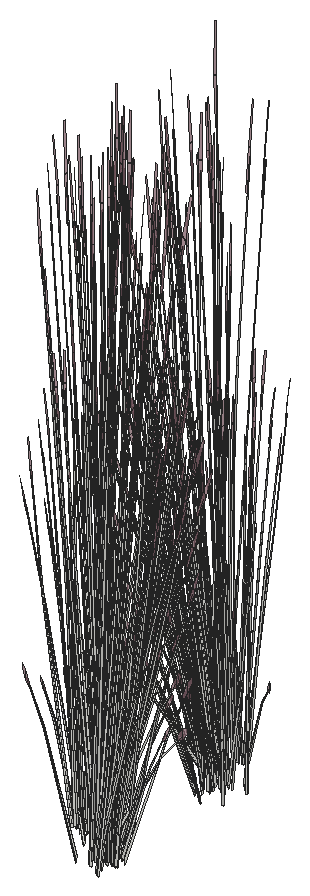
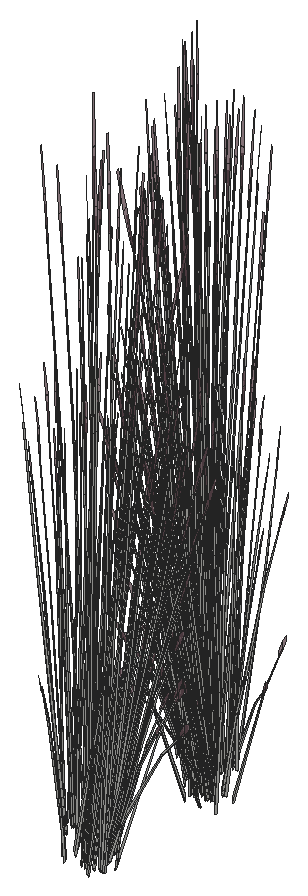
# SketchUp Ruby script. Lengths in inches.
U = 1.inch
M = Sketchup.active_model
def pt(a) = Geom::Point3d.new(a.map { |v| v * U })
def face(e, loops, mat)
  f = e.add_face(loops[0].map { |a| pt(a) })
  loops[1..].each { |l| e.add_face(l.map { |a| pt(a) }).erase! }
  f.material = f.back_material = mat if mat
  f
end
# faces: each face lists its corners as indices into pts; further lists are holes
def faces(e, pts, list, mat = nil) = list.each { |f| face(e, (f[0].is_a?(Array) ? f : [f]).map { |l| l.map { |i| pts[i] } }, mat) }
# xy, xz, yz: faces in a plane at the given z, y or x. An outline is a flat list of corners, or four numbers for a rectangle; further outlines are holes
def ring(l) = l.size == 4 ? [[l[0], l[1]], [l[2], l[1]], [l[2], l[3]], [l[0], l[3]]] : l.each_slice(2).to_a
def flat(e, list, mat, &to3) = list.each { |f| face(e, (f[0].is_a?(Array) ? f : [f]).map { |l| ring(l).map { |u, v| to3.(u, v) } }, mat) }
def xy(e, z, list, mat = nil) = flat(e, list, mat) { |x, y| [x, y, z] }
def xz(e, y, list, mat = nil) = flat(e, list, mat) { |x, z| [x, y, z] }
def yz(e, x, list, mat = nil) = flat(e, list, mat) { |y, z| [x, y, z] }
def lines(e, pts, list) = list.each { |a, b| e.add_line(pt(pts[a]), pt(pts[b])) }
# prism: a flat outline (further loops are holes) pulled along v
def prism(e, loops, v, mat = nil)
  f = face(e, loops, mat); d = Geom::Vector3d.new(v.map { |x| x * U })
  f.pushpull(f.normal.samedirection?(d) ? d.length : -d.length)
end
def box(e, o, s, mat = nil) = prism(e, [[o, [o[0] + s[0], o[1], o[2]], [o[0] + s[0], o[1] + s[1], o[2]], [o[0], o[1] + s[1], o[2]]]], [0, 0, s[2]], mat)
def at(x, y, z, deg = 0) = Geom::Transformation.translation(pt([x, y, z])) * Geom::Transformation.rotation(ORIGIN, Z_AXIS, deg.degrees)
def axes(o, x, y, z) = Geom::Transformation.new([*x, 0, *y, 0, *z, 0, *pt(o).to_a, 1])
def part(name) = M.definitions.add(name)
# library, detail: a bought-in or finely detailed component or shape, given as its bounding box
def library(name, o, s) = part(name).tap { |d| box(d.entities, o, s) }
def detail(e, o, s) = box(e.add_group.entities, o, s)
def put(e, d, t, mat = nil) = e.add_instance(d, t).tap { |i| i.material = mat if mat }
def group(e, t, mat = nil) = e.add_group.tap { |g| g.transformation = t; g.material = mat if mat }.entities
root = M.entities
M.materials.add("LightPink_Translucent").color = [144, 107, 117]
M.materials["LightPink_Translucent"].alpha = 0.75
c1 = part("blade")
p = [[2.15,0.21,22],[0,0.17,0],[0.09,0.45,0],[2.18,0.31,22],[2.29,0.31,22],[0.38,0.45,0],
  [2.48,0.24,33],[2.49,0.24,33],[2.48,0.22,33]]
faces(c1.entities,p,[[0,1,2,3],[4,5,2,3],[6,3,4,7],[8,0,3,6]])
c2 = part("seeds")
p = [[0.3,-0.1,1.38],[-0.01,-0.03,1.59],[-0.01,-0.03,0.03],[0.14,-0.07,-0.07],[0.29,-0.03,3],[0.15,0.01,3.11]]
faces(c2.entities,p,[[0,1,2,3],[1,0,4,5]],"LightPink_Translucent")
c3 = part("blade with seeds")
put(c3.entities,c1,at(0,0,0))
put(c3.entities,c2,axes([2.4,0.25,30.99],[1.5799,-0.05474,1.17369],[-0.12525,1.92788,0.29478],[-0.07173,-0.02425,1.56792]))
put(root,c3,axes([329.36,454.8,1399.49],[0.00895,0.0735,1.76342],[-0.18044,0.38382,-0.26939],[-0.12817,-0.01935,0.30037]))
put(root,c3,axes([331.25,454.39,1400.72],[-0.21202,-0.39143,0.44739],[0.32115,-0.27564,-0.21531],[0.06861,0.04843,1.43643]))
put(root,c3,axes([330.15,456.18,1400.03],[-0.08291,-0.40636,-0.30978],[0.32928,-0.11539,0.30978],[-0.06638,-0.04686,1.38974]))
put(root,c3,axes([330.58,456.16,1400.47],[0.37926,-0.12378,0.17642],[0.09365,0.46065,0.35086],[-0.03382,-0.06712,1.60407]))
put(root,c3,axes([331.36,454.42,1400.67],[0.35635,-0.30962,-0.29095],[0.23697,0.43749,-0.50002],[0.08792,0.04443,1.59708]))
put(root,c3,axes([332.78,455.23,1402.53],[0.29332,0.1301,-0.35414],[-0.08555,0.37955,0.4572],[0.11809,-0.0348,0.87481]))
put(root,c3,axes([330.0625,456.36,1400.02],[-0.33032,-0.23318,-0.49651],[0.19744,-0.41812,0],[-0.07523,-0.05311,1.57504]))
put(root,c3,axes([332.26,453.59,1400.02],[0.33032,0.23318,-0.49651],[-0.19744,0.41812,0],[0.07523,0.05311,1.57504]))
put(root,c3,axes([329.33,454.63,1402.53],[-0.29332,-0.1301,-0.35414],[0.08555,-0.37955,0.4572],[-0.11809,0.0348,0.87481]))
put(root,c3,axes([331.63,454.92,1400.21],[0.39487,0,0],[0,0.48281,0],[0,0,1.78407]))
put(root,c3,axes([330.96,455.53,1400.67],[-0.35635,0.30962,-0.29095],[-0.23697,-0.43749,-0.50002],[-0.08792,-0.04443,1.59708]))
put(root,c3,axes([331.74,453.79,1400.47],[-0.37926,0.12378,0.17642],[-0.09365,-0.46065,0.35086],[0.03382,0.06712,1.60407]))
put(root,c3,axes([331.98,454.76,1401.875],[-0.14639,0.01056,1.71376],[0.09712,-0.45778,0.13857],[0.20862,0.02831,0.73262]))
put(root,c3,axes([332.17,453.77,1400.03],[0.08291,0.40636,-0.30978],[-0.32928,0.11539,0.30978],[0.06638,0.04686,1.38974]))
put(root,c3,axes([332.73,455.39,1402.73],[0.12963,0.31798,0.0643],[-0.23638,0.15564,0.50621],[0.1042,-0.03071,0.77189]))
put(root,c3,axes([331.5,454.68,1400.38],[-0.44609,-0.09826,0.49198],[0.09078,-0.55493,0.19306],[0.06519,0.05359,1.70813]))
put(root,c3,axes([332.71,455.28,1402.73],[-0.09971,0.42522,0.48003],[-0.32782,-0.1454,0.3958],[0.12892,-0.02555,0.9933]))
put(root,c3,axes([331.15,456.05,1400.2],[-0.11516,-0.40207,0],[0.32884,-0.1408,0],[0,0,1.54371]))
put(root,c3,axes([330.93,455.67,1400.62],[-0.06809,0.4162,0.1448],[-0.33266,-0.07225,-0.41347],[-0.06054,-0.04274,1.26744]))
put(root,c3,axes([329.64,454.59,1403.05],[0.29332,0.1301,0.35414],[-0.08555,0.37955,-0.4572],[-0.11809,0.0348,0.87481]))
put(root,c3,axes([331.58,455.99,1400.18],[0.37054,-0.15823,-0.19198],[0.1302,0.45581,0.00008],[0.0409,-0.01749,1.73897]))
put(root,c3,axes([331.71,456.18,1400.47],[0.10196,-0.46348,0.17642],[0.3731,0.13116,0.35086],[-0.06445,0.00226,1.60407]))
put(root,c3,axes([331.62,455.13,1400.21],[0.24637,0.30123,0],[-0.24637,0.30123,0],[0,0,1.69266]))
put(root,c3,axes([330.22,454.57,1401.34],[0.10032,-0.06746,1.77064],[0.0346,0.47103,0.13857],[-0.2173,0.0625,0.63284]))
put(root,c3,axes([332.29,455,1400.47],[-0.2773,-0.3397,0.17642],[0.27945,-0.32949,0.35086],[-0.03063,0.06937,1.60407]))
put(root,c3,axes([331.78,454.49,1400.06],[0.36714,0.07646,-0.62353],[-0.07747,0.47163,-0.16365],[0.10956,0.05715,1.37633]))
put(root,c3,axes([333.4,455.3125,1400.77],[-0.21807,0.07699,1.1486],[0.10265,-0.31819,0.84392],[0.11568,0.02177,0.25299]))
put(root,c3,axes([331.07,456.23,1400.2],[-0.35581,-0.20937,0],[0.17124,-0.43505,0],[0,0,1.62707]))
put(root,c3,axes([331.36,455.67,1400.46],[-0.34464,-0.37536,-0.25192],[0.29,-0.42149,0.5513],[-0.0928,0.04391,1.68216]))
put(root,c3,axes([330.45,456.39,1400.48],[0.33032,0.23318,0.49651],[-0.19744,0.41812,0],[-0.07523,-0.05311,1.57504]))
put(root,c3,axes([331.62,454.78,1400.72],[0.17124,-0.42022,0.44739],[0.35581,0.20224,-0.21531],[0,0.09687,1.43643]))
put(root,c3,axes([333.3,456.66,1402.71],[-0.03191,-0.04083,1.77383],[0.06981,-0.43764,-0.16761],[0.12571,-0.02796,0.31391]))
put(root,c3,axes([329.14,454.88,1402.72],[-0.05763,0.06055,1.74944],[0.0049,0.44239,-0.27667],[-0.13211,0.05753,0.14031]))
put(root,c3,axes([331.55,455.02,1400.29],[0,0.53934,-0.05637],[-0.44133,0,0],[0,0.01695,1.79368]))
put(root,c3,axes([329.53,454.82,1402.68],[-0.09562,0.42421,-0.51099],[-0.32782,-0.1454,-0.3958],[-0.13199,0.0389,0.97773]))
put(root,c3,axes([329.51,454.46,1403.03],[0.17758,0.42229,-0.1216],[-0.31518,0.20752,-0.67495],[-0.13282,0.05572,1.02557]))
put(root,c3,axes([331.58,454.64,1400.21],[0.21202,0.39143,-0.44739],[-0.32115,0.27564,0.21531],[0.06861,0.04843,1.43643]))
put(root,c3,axes([333.02,456.29,1401.93],[-0.06755,-0.39203,-0.03492],[0.31928,-0.09013,-0.15832],[0.06667,0.02485,0.52218]))
put(root,c3,axes([330.26,456.64,1400.375],[-0.22066,0.46731,0],[-0.36918,-0.26061,-0.51607],[-0.08408,-0.05936,1.63711]))
put(root,c3,axes([332.19,456.28,1403.03],[0.0189,-0.47427,-0.1216],[0.35781,0.01296,-0.67495],[0.13781,0.03295,1.02557]))
put(root,c3,axes([332.52,455.01,1400.48],[0,-0.46636,0.49651],[0.39487,0,0],[0,0.10622,1.57504]))
put(root,c3,axes([331.53,455.36,1400.72],[0.38326,-0.02879,0.44739],[0.03466,0.47788,-0.21531],[-0.06861,0.04843,1.43643]))
put(root,c3,axes([331.77,454.875,1400.62],[0.32884,-0.136,0.1448],[0.11516,0.38837,-0.41347],[0,0.08547,1.26744]))
put(root,c3,axes([332.14,456.09,1403.05],[-0.20082,-0.29199,0.35414],[0.2293,-0.2764,-0.4572],[0.1165,0.04206,0.87481]))
put(root,c3,axes([331.1875,455.59,1400.21],[-0.38326,0.02879,-0.44739],[-0.03466,-0.47788,0.21531],[-0.06861,0.04843,1.43643]))
put(root,c3,axes([332.99,455.82,1400.59],[-0.085,-0.1147,1.43002],[0.1106,-0.37943,-0.30754],[0.17198,0.0514,0.61141]))
put(root,c3,axes([331.47,456.24,1400.2],[0.35581,0.20937,0],[-0.17124,0.43505,0],[0,0,1.74954]))
put(root,c3,axes([332.5,456,1402.72],[0.07571,-0.00789,1.74944],[0.20767,-0.36231,-0.27667],[0.13467,0.04783,0.14031]))
put(root,c3,axes([331.61,456.7,1400.19],[-0.21791,-0.46895,-0.05142],[0.36918,-0.26061,0.51607],[-0.09097,0.04465,1.6363]))
put(root,c3,axes([331.53,455.57,1400.62],[0.26075,0.2802,0.1448],[-0.2175,0.31612,-0.41347],[-0.06054,0.04274,1.26744]))
put(root,c3,axes([329.47,455.64,1402.73],[-0.08753,-0.42921,0.48003],[0.34336,-0.07449,0.3958],[-0.1012,0.10094,0.9933]))
put(root,c3,axes([329.41,455.56,1402.73],[-0.2423,-0.19613,0.0643],[0.14107,-0.2793,0.50621],[-0.07768,0.0903,0.77189]))
put(root,c3,axes([329.52,455.04,1401.875],[0.12246,-0.09864,1.71376],[0.1031,0.45582,0.13857],[-0.19225,0.10302,0.73262]))
put(root,c3,axes([332.21,456.05,1402.98],[0.35281,0.01123,-0.71045],[-0.0237,0.47284,0.08574],[0.14947,0.0499,1.00501]))
put(root,c3,axes([331.8125,456.43,1400.48],[0.33032,-0.23318,0.49651],[0.19744,0.41812,0],[-0.07523,0.05311,1.57504]))
put(root,c3,axes([331.34,456.0625,1400.29],[0.15345,0.53576,-0.06012],[-0.43845,0.18773,0],[0.00536,0.01871,1.72173]))
put(root,c3,axes([331.51,456.64,1400.03],[-0.32928,-0.11539,-0.30978],[0.08291,-0.40636,0.30978],[-0.06638,0.04686,1.38974]))
put(root,c3,axes([329.14,455.82,1400.59],[0.12266,0.03828,1.43002],[0.07906,0.39104,-0.30754],[-0.16661,0.0732,0.61141]))
put(root,c3,axes([329.6875,455.5,1403.05],[0.30722,-0.06665,0.35414],[0.08112,0.381,-0.4572],[-0.08804,0.10234,0.87481]))
put(root,c3,axes([332.78,455.09,1400.375],[0.44133,0,0],[0,0.52122,-0.51607],[0,0.11871,1.63711]))
put(root,c3,axes([328.5,455.33,1402.71],[0.04504,0.01251,1.77383],[0.13934,0.41205,-0.16761],[-0.0922,0.10815,0.31391]))
put(root,c3,axes([332.61,455.36,1400.2],[-0.44111,-0.00373,-0.04976],[0,-0.52122,0.49943],[-0.01386,0.11865,1.58352]))
put(root,c3,axes([331.65,454.91,1400.67],[0.39748,0.22252,-0.29095],[-0.19139,0.46966,-0.50002],[0.01249,0.11531,1.59708]))
put(root,c3,axes([328.88,456.64,1400.77],[0.14709,-0.21136,1.1486],[0.05804,0.3346,0.84392],[-0.1063,0.05991,0.25299]))
put(root,c3,axes([332.42,456.25,1402.53],[0.20082,0.29199,-0.35414],[-0.2293,0.2764,0.4572],[0.1165,0.04206,0.87481]))
put(root,c3,axes([332.52,455.4375,1400.03],[-0.24637,0.29097,-0.30978],[-0.24637,-0.29097,0.30978],[0,0.09372,1.38974]))
put(root,c3,axes([331.46,455.46,1400.67],[0.04113,0.53214,-0.29095],[-0.42835,0.03218,-0.50002],[-0.07543,0.07088,1.59708]))
put(root,c3,axes([332.32,456.36,1402.73],[-0.01777,0.35463,0.0643],[-0.26836,-0.00972,0.50621],[0.1028,0.03711,0.77189]))
put(root,c3,axes([331.61,455.26,1400.21],[-0.17124,0.42022,-0.44739],[-0.35581,-0.20224,0.21531],[0,0.09687,1.43643]))
put(root,c3,axes([329.43,455.72,1402.53],[-0.30722,0.06665,-0.35414],[-0.08112,-0.381,0.4572],[-0.08804,0.10234,0.87481]))
put(root,c3,axes([332.34,456.25,1402.73],[-0.26024,0.30729,0.48003],[-0.22444,-0.32634,0.3958],[0.1221,0.05668,0.9933]))
put(root,c3,axes([328.99,456.58,1403.65],[0.31145,0.12449,-0.06488],[-0.0958,0.38314,-0.29416],[-0.05094,0.05817,0.97024]))
put(root,c3,axes([331.2,455.87,1400.06],[-0.23773,0.35053,-0.62353],[-0.29532,-0.31785,-0.16365],[-0.09526,0.08744,1.37633]))
put(root,c3,axes([331.52,456.6,1403.05],[-0.05451,-0.37564,0.35414],[0.31161,-0.09919,-0.4572],[0.0837,0.10765,0.87481]))
put(root,c3,axes([331.62,456.46,1400.33],[0.44186,0.15158,0.30756],[-0.11054,0.54181,-0.36492],[-0.07313,0.06781,1.64885]))
put(root,c3,axes([331.59,456.83,1400.02],[-0.33032,0.23318,-0.49651],[-0.19744,-0.41812,0],[-0.07523,0.05311,1.57504]))
put(root,c3,axes([332.6875,455.45,1400.02],[0,0.46636,-0.49651],[-0.39487,0,0],[0,0.10622,1.57504]))
put(root,c3,axes([331.7,455.5,1401.875],[-0.1311,-0.08035,1.71376],[0.27131,-0.33708,0.13857],[0.16909,0.15206,0.73262]))
put(root,c3,axes([331.72,454.44,1402.47],[-0.30498,-0.24231,1.38283],[0.32203,-0.37727,0.59665],[0.0984,0.22736,1.33663]))
put(root,c3,axes([329.53,455.46,1403.03],[0.32648,0.25715,-0.1216],[-0.18809,0.3724,-0.67495],[-0.09224,0.12945,1.02557]))
put(root,c3,axes([332.18,456.41,1400.77],[-0.19872,-0.13409,1.1486],[0.2566,-0.13625,0.84392],[0.06921,0.11541,0.25299]))
put(root,c3,axes([331.49,456.8,1403.03],[0.21031,-0.39918,-0.1216],[0.30457,0.22997,-0.67495],[0.10587,0.11278,1.02557]))
put(root,c3,axes([329.97,455.35,1401.875],[0.08815,-0.14329,1.71376],[0.22258,0.38678,0.13857],[-0.15267,0.17614,0.73262]))
put(root,c3,axes([329.6875,455.77,1402.68],[0.09067,0.42583,-0.51099],[-0.34336,0.07449,-0.3958],[-0.0984,0.11438,0.97773]))
put(root,c3,axes([330.1,456.26,1403.05],[0.23881,-0.24554,0.35414],[0.22606,0.28036,-0.4572],[-0.0344,0.14245,0.87481]))
put(root,c3,axes([331.89,456.75,1400.375],[0.22066,0.46731,0],[-0.36918,0.26061,-0.51607],[-0.08408,0.05936,1.63711]))
put(root,c3,axes([331.21,457.13,1402.71],[0.00104,-0.05646,1.77383],[0.30246,-0.2491,-0.16761],[0.10506,0.08891,0.31391]))
put(root,c3,axes([332.24,456.91,1399.49],[0.02571,-0.06733,1.76342],[0.32373,-0.19829,-0.26939],[0.09815,0.10263,0.30037]))
put(root,c3,axes([331.7,454.9,1400.84],[-0.00964,-0.43909,1.41272],[0.43635,0.11382,0.59816],[-0.1032,0.24027,1.3335]))
put(root,c3,axes([331.8125,455.38,1400.09],[0.12941,0.42699,-0.69212],[-0.37279,0.15378,-0.18165],[0.0143,0.14459,1.52773]))
put(root,c3,axes([329.88,456.48,1402.73],[-0.29004,-0.02173,0.0643],[0.00795,-0.32812,0.50621],[-0.03035,0.12569,0.77189]))
put(root,c3,axes([329.27,456.85,1399.49],[0.04734,0.04659,1.76342],[0.08027,0.4317,-0.26939],[-0.10492,0.09206,0.30037]))
put(root,c3,axes([329.98,456.51,1402.73],[-0.25132,-0.3182,0.48003],[0.2669,-0.27442,0.3958],[-0.04636,0.14929,0.9933]))
put(root,c3,axes([331.74,456.6,1402.68],[0.34827,-0.11086,-0.51099],[0.06092,0.41983,-0.3958],[0.09354,0.12031,0.97773]))
put(root,c3,axes([330.77,456.66,1403.05],[0.1064,-0.35863,0.35414],[0.31043,0.1046,-0.4572],[0.02846,0.14439,0.87481]))
put(root,c3,axes([332.22,457.02,1400.67],[-0.22633,-0.01463,1.0506],[0.14947,-0.31064,0.58006],[0.08941,0.11036,0.8241]))
put(root,c3,axes([331.56,456.94,1402.73],[-0.16041,0.29625,0.0643],[-0.22843,-0.17248,0.50621],[0.07385,0.09498,0.77189]))
put(root,c3,axes([331.1875,457.94,1403.65],[0.2439,-0.26754,-0.06488],[0.22348,0.29302,-0.29416],[0.01573,0.08303,0.97024]))
put(root,c3,axes([331.63,456.86,1402.73],[-0.35104,0.10702,0.48003],[-0.06092,-0.41983,0.3958],[0.08256,0.12373,0.9933]))
put(root,c3,axes([329.9,455.7,1401.875],[0.06572,-0.16029,1.71376],[0.27569,0.33172,0.13857],[-0.12437,0.20675,0.73262]))
put(root,c3,axes([331.48,456.27,1400.59],[0.00623,-0.15459,1.43002],[0.29764,-0.17268,-0.30754],[0.09188,0.18503,0.61141]))
put(root,c3,axes([330.67,456.99,1402.73],[-0.26007,0.1585,0.0643],[-0.12729,-0.28902,0.50621],[0.02512,0.1274,0.77189]))
put(root,c3,axes([329.98,456.61,1402.53],[-0.23881,0.24554,-0.35414],[-0.22606,-0.28036,0.4572],[-0.0344,0.14245,0.87481]))
put(root,c3,axes([329.15,456.53,1402.72],[-0.00877,0.09229,1.74944],[0.24897,0.32105,-0.27667],[-0.06518,0.15182,0.14031]))
put(root,c3,axes([329.95,456.32,1403.4],[0.3879,0.02311,-0.13498],[-0.0106,0.43749,-0.74919],[-0.02694,0.1685,1.13838]))
put(root,c3,axes([330.67,456.8125,1403.03],[0.34538,-0.21713,-0.1216],[0.16972,0.38536,-0.67495],[0.04557,0.16239,1.02557]))
put(root,c3,axes([330.77,456.96,1403.0625],[-0.34777,-0.12192,0.53283],[0.11892,-0.40083,0.43934],[0.0209,0.15763,1.10256]))
put(root,c3,axes([330.13,457.56,1400.77],[-0.00913,-0.2773,1.1486],[0.22824,0.19778,0.84392],[-0.04489,0.13217,0.25299]))
put(root,c3,axes([330.73,456.9,1399.49],[0.05712,-0.02538,1.76342],[0.34359,0.13968,-0.26939],[0.01005,0.15742,0.30037]))
put(root,c3,axes([330.21,456.49,1403],[0.25266,0.31335,-0.5672],[-0.2669,0.27442,-0.43934],[-0.03844,0.15921,1.08528]))
put(root,c3,axes([329.9375,456.96,1400.82],[0.32063,-0.08258,0.06507],[0.07371,0.33271,-0.86304],[-0.02033,0.16842,0.7736]))
put(root,c3,axes([330.96,456.79,1402.68],[0.34695,0.11691,-0.51099],[-0.11892,0.40083,-0.3958],[0.03181,0.16138,0.97773]))
put(root,c3,axes([331.16,455.97,1401.875],[-0.08068,-0.14973,1.71376],[0.3728,-0.12606,0.13857],[0.08426,0.23506,0.73262]))
put(root,c3,axes([330.8,457.04,1402.53],[-0.1064,0.35863,-0.35414],[-0.31043,-0.1046,0.4572],[0.02846,0.14439,0.87481]))
put(root,c3,axes([330.13,456.35,1403.34],[-0.00918,0.43138,-0.7886],[-0.38672,-0.02897,0.09517],[-0.04081,0.18275,1.11556]))
put(root,c3,axes([329.125,457.48,1402.71],[0.04004,-0.02816,1.77383],[0.33095,0.18728,-0.16761],[-0.00778,0.15594,0.31391]))
put(root,c3,axes([330.5,456.04,1401.875],[-0.00864,-0.17899,1.71376],[0.37441,0.11874,0.13857],[-0.02316,0.25508,0.73262]))
put(root,c3,axes([330.84,456.72,1402.98],[0.16845,0.3792,-0.71045],[-0.34676,0.21133,0.08574],[0.03939,0.18322,1.00501]))
put(root,c3,axes([329.86,457.3125,1400.59],[0.11138,-0.07357,1.43002],[0.27499,0.22183,-0.30754],[-0.08185,0.19194,0.61141]))
put(root,c3,axes([330.58,457.67,1402.72],[0.04474,0.0751,1.74944],[0.36104,0.0295,-0.27667],[0.03631,0.16562,0.14031]))
put(root,c3,axes([330.01,456.95,1401.36],[0.00775,-0.24075,1.54345],[0.34877,0.12716,0.21329],[-0.03022,0.25658,0.72882]))
put(root,c3,axes([330.27,468.32,1401.875],[0.08068,0.14973,1.71376],[-0.3728,0.12606,0.13857],[-0.08426,-0.23506,0.73262]))
put(root,c3,axes([330.89,467.32,1402.72],[-0.05398,-0.06539,1.74944],[-0.36026,0.04145,-0.27667],[-0.0575,-0.15639,0.14031]))
put(root,c3,axes([331.72,468.1,1400.59],[-0.10032,0.0944,1.43002],[-0.30046,-0.16522,-0.30754],[0.05569,-0.20547,0.61141]))
put(root,c3,axes([331.27,468.43,1402.98],[-0.16845,-0.3792,-0.71045],[0.34676,-0.21133,0.08574],[-0.03939,-0.18322,1.00501]))
put(root,c3,axes([330.17,467.92,1400.59],[-0.02137,0.15256,1.43002],[-0.31245,0.12771,-0.30754],[-0.07303,-0.19719,0.61141]))
put(root,c3,axes([330.98,467.59,1399.49],[-0.0592,0.0168,1.76342],[-0.32738,-0.18913,-0.26939],[0.00549,-0.15776,0.30037]))
put(root,c3,axes([331.97,468.8,1402.98],[0.00918,-0.43138,-0.71045],[0.38672,0.02897,0.08574],[0.04081,-0.18275,1.00501]))
put(root,c3,axes([332.51,468.125,1402.72],[-0.00341,-0.09282,1.74944],[-0.28775,-0.26825,-0.27667],[0.04449,-0.16261,0.14031]))
put(root,c3,axes([331.3,468.11,1402.53],[0.1064,-0.35863,-0.35414],[0.31043,0.1046,0.4572],[-0.02846,-0.14439,0.87481]))
put(root,c3,axes([331.53,468.58,1401.875],[-0.06572,0.16029,1.71376],[-0.27569,-0.33172,0.13857],[0.12437,-0.20675,0.73262]))
put(root,c3,axes([332.43,467.79,1402.71],[-0.03584,0.03562,1.77383],[-0.35118,-0.12018,-0.16761],[-0.01271,-0.15545,0.31391]))
put(root,c3,axes([331.14,468.35,1402.68],[-0.34695,-0.11691,-0.51099],[0.11892,-0.40083,-0.3958],[-0.03181,-0.16138,0.97773]))
put(root,c3,axes([331.35,467.35,1400.77],[0.04528,0.27194,1.1486],[-0.25117,-0.15062,0.84392],[0.02703,-0.13924,0.25299]))
put(root,c3,axes([331.89,468.66,1402.68],[-0.25266,-0.31335,-0.51099],[0.2669,-0.27442,-0.3958],[0.03844,-0.15921,0.97773]))
put(root,c3,axes([330.52,467.11,1402.71],[-0.00658,0.0559,1.77383],[-0.32474,0.20287,-0.16761],[-0.09556,-0.1037,0.31391]))
put(root,c3,axes([330.45,468.1,1403.09],[0.39316,-0.11987,0.53763],[0.06823,0.47021,0.4433],[-0.09247,-0.13858,1.11249]))
put(root,c3,axes([331.34,468.19,1402.73],[0.34777,0.12192,0.48003],[-0.11892,0.40083,0.3958],[-0.0209,-0.15763,0.9933]))
put(root,c3,axes([331.4375,468.33,1403.03],[-0.34538,0.21713,-0.1216],[-0.16972,-0.38536,-0.67495],[-0.04557,-0.16239,1.02557]))
put(root,c3,axes([332.15,468.82,1403.03],[-0.3879,-0.02311,-0.1216],[0.0106,-0.43749,-0.67495],[0.02694,-0.1685,1.02557]))
put(root,c3,axes([332.13,468.54,1402.53],[0.23881,-0.24554,-0.35414],[0.22606,0.28036,0.4572],[0.0344,-0.14245,0.87481]))
put(root,c3,axes([330.0625,467.68,1400.77],[0.18411,0.16231,1.1486],[-0.26813,0.09757,0.84392],[-0.05737,-0.12474,0.25299]))
put(root,c3,axes([331.43,468.16,1402.73],[0.26007,-0.1585,0.0643],[0.12729,0.28902,0.50621],[-0.02512,-0.1274,0.77189]))
put(root,c3,axes([330.51,468.54,1402.98],[-0.30095,-0.22541,-0.71045],[0.21388,-0.395,0.08574],[-0.10904,-0.13459,1.00501]))
put(root,c3,axes([330.4,468.24,1402.53],[-0.05451,-0.37564,-0.35414],[0.31161,-0.09919,0.4572],[-0.0837,-0.10765,0.87481]))
put(root,c3,axes([330.54,468.2,1402.73],[0.16041,-0.29625,0.0643],[0.22843,0.17248,0.50621],[-0.07385,-0.09498,0.77189]))
put(root,c3,axes([329.92,468.16,1399.49],[-0.03419,0.06144,1.76342],[-0.3455,0.13246,-0.26939],[-0.08346,-0.12049,0.30037]))
put(root,c3,axes([330.49,469.85,1400.1],[-0.14494,-0.47823,-0.69835],[0.41752,-0.17223,-0.18329],[-0.01602,-0.16194,1.54149]))
put(root,c3,axes([329.73,468.78,1401.875],[0.1311,0.08035,1.71376],[-0.27131,0.33708,0.13857],[-0.16909,-0.15206,0.73262]))
put(root,c3,axes([332.43,468.39,1399.49],[-0.05283,-0.03674,1.76342],[-0.13569,-0.41045,-0.26939],[0.09154,-0.11138,0.30037]))
put(root,c3,axes([331.33,468.48,1403.05],[-0.1064,0.35863,0.35414],[-0.31043,-0.1046,-0.4572],[-0.02846,-0.14439,0.87481]))
put(root,c3,axes([330.37,468.55,1402.68],[-0.34827,0.11086,-0.51099],[-0.06092,-0.41983,-0.3958],[-0.09354,-0.12031,0.97773]))
put(root,c3,axes([332.125,468.64,1402.73],[0.25132,0.3182,0.48003],[-0.2669,0.27442,0.3958],[0.04636,-0.14929,0.9933]))
put(root,c3,axes([330.61,468.17,1403.43],[-0.23555,0.44708,-0.13619],[-0.34112,-0.25757,-0.75594],[-0.11858,-0.12631,1.14864]))
put(root,c3,axes([332.22,468.67,1402.73],[0.29004,0.02173,0.0643],[-0.00795,0.32812,0.50621],[0.03035,-0.12569,0.77189]))
put(root,c3,axes([332,468.89,1403.05],[-0.23881,0.24554,0.35414],[-0.22606,-0.28036,-0.4572],[0.0344,-0.14245,0.87481]))
put(root,c3,axes([332.42,469.55,1402.98],[0.18436,-0.36797,-0.71045],[0.32306,0.26151,0.08574],[0.11008,-0.13332,1.00501]))
put(root,c3,axes([330.43,468.48,1400.375],[-0.22066,-0.46731,0],[0.36918,-0.26061,-0.51607],[0.08408,-0.05936,1.63711]))
put(root,c3,axes([332.41,469.38,1402.68],[-0.09067,-0.42583,-0.51099],[0.34336,-0.07449,-0.3958],[0.0984,-0.11438,0.97773]))
put(root,c3,axes([330.92,467.91,1400.13],[-0.2439,0.26754,-0.03893],[-0.22348,-0.29302,-0.17649],[-0.01573,-0.08303,0.58215]))
put(root,c3,axes([329.71,468.04,1402.72],[-0.07594,-0.00329,1.74944],[-0.24177,0.32918,-0.27667],[-0.129,-0.06726,0.14031]))
put(root,c3,axes([332.58,469.68,1403.03],[-0.32648,-0.25715,-0.1216],[0.18809,-0.3724,-0.67495],[0.09224,-0.12945,1.02557]))
put(root,c3,axes([331.23,471.09,1401.33],[0.305,0.18805,1.51261],[-0.29879,0.40513,0.59816],[-0.13384,-0.24012,1.26806]))
put(root,c3,axes([330.59,468.54,1403.05],[0.05451,0.37564,0.35414],[-0.31161,0.09919,-0.4572],[-0.0837,-0.10765,0.87481]))
put(root,c3,axes([329.63,469.79,1400.02],[0,-0.46636,-0.49651],[0.39487,0,0],[0,-0.10622,1.57504]))
put(root,c3,axes([330.73,468.41,1400.02],[0.33032,-0.23318,-0.49651],[0.19744,0.41812,0],[0.07523,-0.05311,1.57504]))
put(root,c3,axes([332.69,469.21,1400.59],[-0.12609,-0.01381,1.43002],[-0.12917,-0.37055,-0.30754],[0.1549,-0.10482,0.61141]))
put(root,c3,axes([329.65,468.79,1403.09],[0.29147,-0.34417,0.53763],[0.25138,0.3655,0.4433],[-0.13675,-0.06349,1.11249]))
put(root,c3,axes([333.38,469.57,1402.71],[-0.0461,-0.00354,1.77383],[-0.19143,-0.37951,-0.16761],[0.07688,-0.12478,0.31391]))
put(root,c3,axes([331.12,469.36,1400.06],[0.23773,-0.35053,-0.62353],[0.29532,0.31785,-0.16365],[0.09526,-0.08744,1.37633]))
put(root,c3,axes([332.84,468.53,1400.77],[-0.11756,0.2374,1.1486],[-0.10105,-0.31895,0.84392],[0.09709,-0.07992,0.25299]))
put(root,c3,axes([332.67,469.42,1402.53],[0.30722,-0.06665,-0.35414],[0.08112,0.381,0.4572],[0.08804,-0.10234,0.87481]))
put(root,c3,axes([329.78,468.79,1402.73],[0.01777,-0.35463,0.0643],[0.26836,0.00972,0.50621],[-0.1028,-0.03711,0.77189]))
put(root,c3,axes([330.71,469.98,1400.21],[0.17124,-0.42022,-0.44739],[0.35581,0.20224,0.21531],[0,-0.09687,1.43643]))
put(root,c3,axes([329.68,468.9,1402.53],[-0.20082,-0.29199,-0.35414],[0.2293,-0.2764,0.4572],[-0.1165,-0.04206,0.87481]))
put(root,c3,axes([330.86,469.77,1400.67],[-0.04113,-0.53214,-0.29095],[0.42835,-0.03218,-0.50002],[0.07543,-0.07088,1.59708]))
put(root,c3,axes([329.8,469.8,1400.03],[0.24637,-0.29097,-0.30978],[0.24637,0.29097,0.30978],[0,-0.09372,1.38974]))
put(root,c3,axes([329.7,468.4,1400.13],[-0.10181,0.3808,-0.03893],[-0.31336,-0.11714,-0.17649],[-0.04758,-0.06228,0.58215]))
put(root,c3,axes([332.42,469.65,1403.05],[-0.30722,0.06665,0.35414],[-0.08112,-0.381,-0.4572],[0.08804,-0.10234,0.87481]))
put(root,c3,axes([330.67,470.33,1400.67],[-0.39748,-0.22252,-0.29095],[0.19139,-0.46966,-0.50002],[-0.01249,-0.11531,1.59708]))
put(root,c3,axes([329.53,470.14,1400.375],[-0.44133,0,0],[0,-0.52122,-0.51607],[0,-0.11871,1.63711]))
put(root,c3,axes([329.61,469.21,1400.59],[0.06891,0.12984,1.43002],[-0.15879,0.35293,-0.30754],[-0.16304,-0.08436,0.61141]))
put(root,c3,axes([330.81,468.59,1400.03],[0.32928,0.11539,-0.30978],[-0.08291,0.40636,0.30978],[0.06638,-0.04686,1.38974]))
put(root,c3,axes([329.89,469.09,1402.98],[-0.35281,-0.01123,-0.71045],[0.0237,-0.47284,0.08574],[-0.14947,-0.0499,1.00501]))
put(root,c3,axes([332.7,469.59,1402.73],[0.2423,0.19613,0.0643],[-0.14107,0.2793,0.50621],[0.07768,-0.0903,0.77189]))
put(root,c3,axes([332.63,469.5,1402.73],[0.08753,0.42921,0.48003],[-0.34336,0.07449,0.3958],[0.1012,-0.10094,0.9933]))
put(root,c3,axes([333.55,470.02,1402.72],[0.04898,-0.07104,1.74944],[-0.06269,-0.43574,-0.27667],[0.12289,-0.08262,0.14031]))
put(root,c3,axes([329.875,470,1400.33],[-0.32829,0.39208,0.30756],[-0.32849,-0.38796,-0.36492],[-0.01146,-0.11134,1.64885]))
put(root,c3,axes([329.42,468.32,1402.71],[0.02617,0.04654,1.77383],[-0.12614,0.41836,-0.16761],[-0.12775,0.00303,0.31391]))
put(root,c3,axes([330.92,470.19,1400.43],[0.39767,0.22603,0.24065],[-0.19139,0.46966,0.50002],[0,-0.10827,1.60543]))
put(root,c3,axes([330.77,470.82,1400.4375],[0.09355,-0.55261,-0.23429],[0.44354,0.09633,0.51271],[-0.0775,-0.07631,1.5644]))
put(root,c3,axes([329.78,469.1875,1402.68],[-0.25628,0.30892,-0.51099],[-0.22444,-0.32634,-0.3958],[-0.13021,-0.047,0.97773]))
put(root,c3,axes([329.97,469.05,1403.05],[0.20082,0.29199,0.35414],[-0.2293,0.2764,-0.4572],[-0.1165,-0.04206,0.87481]))
put(root,c3,axes([329.2,469.6,1400.77],[0.22533,-0.03337,1.1486],[-0.14293,0.29403,0.84392],[-0.11135,-0.04411,0.25299]))
put(root,c3,axes([330.79,469.87,1400.72],[-0.38326,0.02879,0.44739],[-0.03466,-0.47788,-0.21531],[0.06861,-0.04843,1.43643]))
put(root,c3,axes([329.91,468.87,1403.03],[-0.0189,0.47427,-0.1216],[-0.35781,-0.01296,-0.67495],[-0.13781,-0.03295,1.02557]))
put(root,c3,axes([329.8,470.22,1400.48],[0,0.46636,0.49651],[-0.39487,0,0],[0,-0.10622,1.57504]))
put(root,c3,axes([332.59,470.6875,1403.03],[-0.17758,-0.42229,-0.1216],[0.31518,-0.20752,-0.67495],[0.13282,-0.05572,1.02557]))
put(root,c3,axes([332.57,470.32,1402.68],[0.09562,-0.42421,-0.51099],[0.32782,0.1454,-0.3958],[0.13199,-0.0389,0.97773]))
put(root,c3,axes([332.06,468.6,1400.375],[0.22066,-0.46731,0],[0.36918,0.26061,-0.51607],[0.08408,0.05936,1.63711]))
put(root,c3,axes([329.46,469.52,1401.875],[0.14639,-0.01056,1.71376],[-0.09712,0.45778,0.13857],[-0.20862,-0.02831,0.73262]))
put(root,c3,axes([330.73,470.6,1400.21],[-0.21202,-0.39143,-0.44739],[0.32115,-0.27564,0.21531],[-0.06861,-0.04843,1.43643]))
put(root,c3,axes([330.78,470.04,1400.36],[0.15345,0.52148,0.45755],[-0.43845,0.18134,0.17955],[0.00536,-0.09582,1.58856]))
put(root,c3,axes([332.92,470.44,1399.98],[-0.22732,0.05597,1.41583],[-0.03618,-0.44548,0.08104],[0.15921,-0.06743,0.80566]))
put(root,c3,axes([333.34,470.05,1400.26],[-0.21881,-0.29821,-0.06488],[0.23965,-0.27324,-0.29416],[0.0679,-0.01924,0.97024]))
put(root,c3,axes([330.7,470.45,1400.72],[-0.17124,0.42022,0.44739],[-0.35581,-0.20224,-0.21531],[0,-0.09687,1.43643]))
put(root,c3,axes([331.33,470.09,1400.21],[0,-0.53961,0],[0.44133,0,0],[0,0,1.79456]))
put(root,c3,axes([331.87,468.84,1400.48],[-0.33032,-0.23318,0.49651],[0.19744,-0.41812,0],[0.07523,0.05311,1.57504]))
put(root,c3,axes([332.51,470.48,1402.98],[0.31014,-0.20596,-0.71045],[0.17284,0.42397,0.08574],[0.14985,-0.04816,1.00501]))
put(root,c3,axes([330.54,470.75,1400.06],[-0.36714,-0.07646,-0.62353],[0.07747,-0.47163,-0.16365],[-0.10956,-0.05715,1.37633]))
